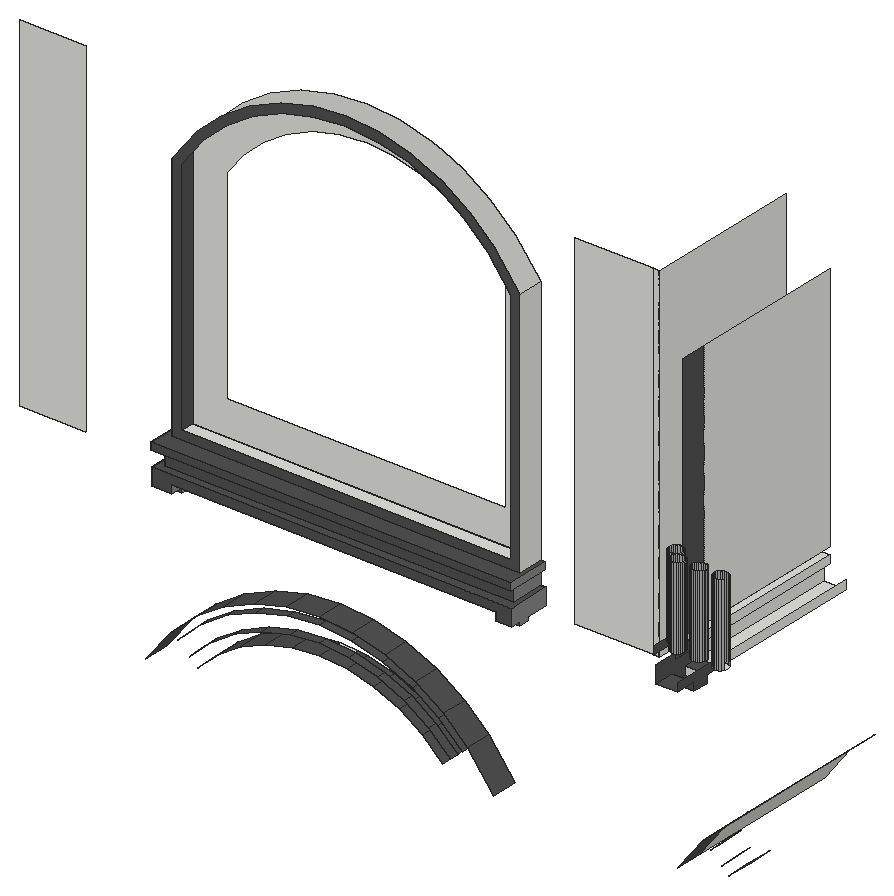
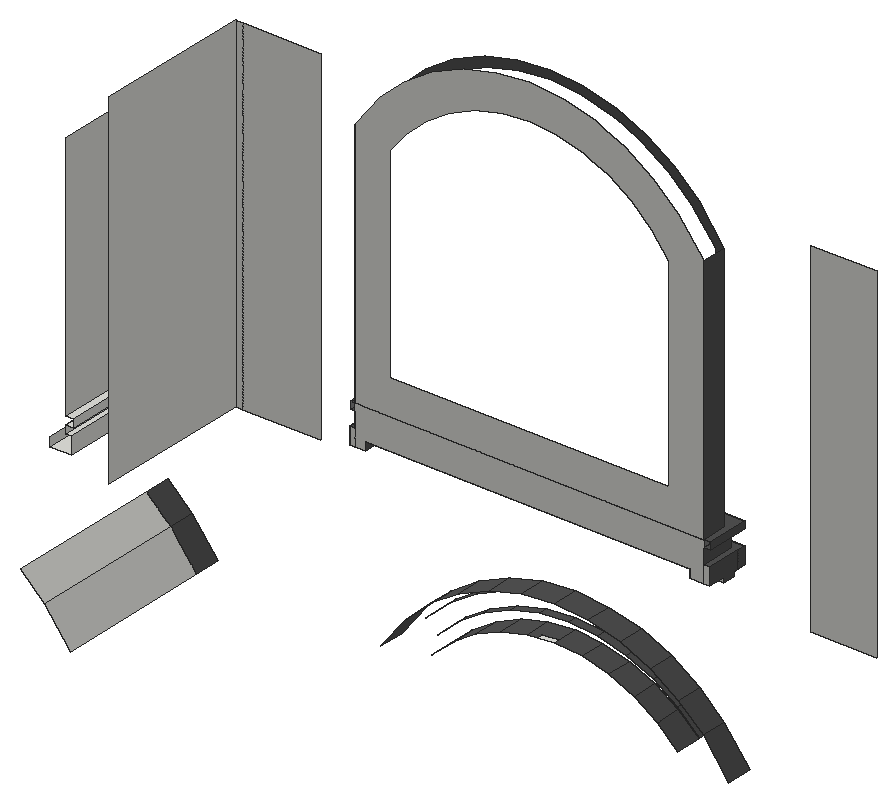
# SketchUp Ruby script. Lengths in inches.
U = 1.inch
M = Sketchup.active_model
def pt(a) = Geom::Point3d.new(a.map { |v| v * U })
def face(e, loops, mat)
  f = e.add_face(loops[0].map { |a| pt(a) })
  loops[1..].each { |l| e.add_face(l.map { |a| pt(a) }).erase! }
  f.material = f.back_material = mat if mat
  f
end
# faces: each face lists its corners as indices into pts; further lists are holes
def faces(e, pts, list, mat = nil) = list.each { |f| face(e, (f[0].is_a?(Array) ? f : [f]).map { |l| l.map { |i| pts[i] } }, mat) }
# xy, xz, yz: faces in a plane at the given z, y or x. An outline is a flat list of corners, or four numbers for a rectangle; further outlines are holes
def ring(l) = l.size == 4 ? [[l[0], l[1]], [l[2], l[1]], [l[2], l[3]], [l[0], l[3]]] : l.each_slice(2).to_a
def flat(e, list, mat, &to3) = list.each { |f| face(e, (f[0].is_a?(Array) ? f : [f]).map { |l| ring(l).map { |u, v| to3.(u, v) } }, mat) }
def xy(e, z, list, mat = nil) = flat(e, list, mat) { |x, y| [x, y, z] }
def xz(e, y, list, mat = nil) = flat(e, list, mat) { |x, z| [x, y, z] }
def yz(e, x, list, mat = nil) = flat(e, list, mat) { |y, z| [x, y, z] }
def lines(e, pts, list) = list.each { |a, b| e.add_line(pt(pts[a]), pt(pts[b])) }
# prism: a flat outline (further loops are holes) pulled along v
def prism(e, loops, v, mat = nil)
  f = face(e, loops, mat); d = Geom::Vector3d.new(v.map { |x| x * U })
  f.pushpull(f.normal.samedirection?(d) ? d.length : -d.length)
end
def box(e, o, s, mat = nil) = prism(e, [[o, [o[0] + s[0], o[1], o[2]], [o[0] + s[0], o[1] + s[1], o[2]], [o[0], o[1] + s[1], o[2]]]], [0, 0, s[2]], mat)
def at(x, y, z, deg = 0) = Geom::Transformation.translation(pt([x, y, z])) * Geom::Transformation.rotation(ORIGIN, Z_AXIS, deg.degrees)
def axes(o, x, y, z) = Geom::Transformation.new([*x, 0, *y, 0, *z, 0, *pt(o).to_a, 1])
def part(name) = M.definitions.add(name)
# library, detail: a bought-in or finely detailed component or shape, given as its bounding box
def library(name, o, s) = part(name).tap { |d| box(d.entities, o, s) }
def detail(e, o, s) = box(e.add_group.entities, o, s)
def put(e, d, t, mat = nil) = e.add_instance(d, t).tap { |i| i.material = mat if mat }
def group(e, t, mat = nil) = e.add_group.tap { |g| g.transformation = t; g.material = mat if mat }.entities
root = M.entities
M.materials.add("[0132_LightGray]").color = [169, 169, 169]
M.materials.add("[0133_Gray]").color = [135, 135, 135]
M.materials.add("[0135_DarkGray]").color = [81, 81, 81]
xy(root,480.35,[[62.57,39.32,69.5625,43.6875]],"[0135_DarkGray]")
xy(root,480.91,[[181.99,38.25,187.51,42]],"[0135_DarkGray]")
xy(root,481.53,[[240.07,38.6875,247.74,44.12]],"[0135_DarkGray]")
xy(root,481.97,[[62.57,34.6875,69.5625,39.32],[181.99,34.6875,187.51,38.25],[181.99,42,187.51,49.6875],[62.57,43.6875,69.5625,49.6875]],"[0135_DarkGray]")
xy(root,484.28,[[240.07,49.6875,247.74,104.375]])
xy(root,484.28,[[240.07,31.6875,247.74,38.6875],[240.07,44.12,247.74,49.6875]],"[0135_DarkGray]")
xy(root,484.97,[[69.5625,34.6875,181.99,49.6875]],"[0135_DarkGray]")
xy(root,487.85,[[62.57,34.6875,187.51,34.6875,187.51,49.6875,185.82,49.6875,185.82,37.6875,64.89,37.6875,64.89,49.6875,62.57,49.6875]],"[0135_DarkGray]")
xy(root,490.18,[[240.07,49.6875,242.14,104.375]])
xy(root,493.07,[[239.45,49.6875,242.14,104.375]])
xy(root,493.17,[[62.39,34.6875,62.39,49.6875,64.89,49.6875,64.89,37.6875,185.82,37.6875,185.82,49.6875,187.14,49.6875,187.14,34.6875]],"[0135_DarkGray]")
xy(root,495.66,[[245.54,31.88,244.91,31.96,244.32,32.21,243.82,32.6,243.43,33.1,243.18,33.6875,243.1,34.32,243.18,34.95,243.43,35.54,243.82,36.04,244.32,36.43,244.91,36.67,245.54,36.76,246.17,36.67,246.76,36.43,247.26,36.04,247.65,35.54,247.89,34.95,247.98,34.32,247.89,33.6875,247.65,33.1,247.26,32.6,246.76,32.21,246.17,31.96],[252.98,31.88,252.35,31.96,251.76,32.21,251.25,32.6,250.87,33.1,250.62,33.6875,250.54,34.32,250.62,34.95,250.87,35.54,251.25,36.04,251.76,36.43,252.35,36.67,252.98,36.76,253.61,36.67,254.2,36.43,254.7,36.04,255.09,35.54,255.33,34.95,255.41,34.32,255.33,33.6875,255.09,33.1,254.7,32.6,254.2,32.21,253.61,31.96],[260.41,31.88,259.78,31.96,259.2,32.21,258.69,32.6,258.3,33.1,258.06,33.6875,257.98,34.32,258.06,34.95,258.3,35.54,258.69,36.04,259.2,36.43,259.78,36.67,260.41,36.76,261.04,36.67,261.63,36.43,262.14,36.04,262.53,35.54,262.77,34.95,262.85,34.32,262.77,33.6875,262.53,33.1,262.14,32.6,261.63,32.21,261.04,31.96],[64.89,40.6875,185.57,49.6875],[239.45,49.6875,242.14,104.375]])
xy(root,495.66,[[62.39,34.6875,187.14,34.6875,187.14,49.6875,185.57,49.6875,185.57,40.6875,64.89,40.6875,64.89,49.6875,62.39,49.6875]],"[0135_DarkGray]")
xz(root,34.6875,[[62.57,481.97,69.5625,481.97,69.5625,484.97,181.99,484.97,181.99,481.97,187.51,481.97,187.51,487.85,62.57,487.85],[62.39,493.17,187.14,495.66]],"[0135_DarkGray]")
xz(root,37.6875,[[64.89,487.85,185.82,493.17]],"[0135_DarkGray]")
xz(root,38.25,[[181.99,480.91,187.51,481.97]],"[0135_DarkGray]")
xz(root,38.6875,[[240.07,481.53,247.74,484.28]],"[0135_DarkGray]")
xz(root,39.32,[[62.57,480.35,69.5625,481.97]],"[0135_DarkGray]")
xz(root,40.6875,[[[64.89,495.66,185.57,495.66,185.57,582.07,176.65,593.68,168.18,601.54,158.52,607.9,151.56,610.98,147.95,612.57,136.75,615.43,125.23,616.39,113.71,615.43,102.51,612.57,98.9,610.98,91.93,607.9,82.28,601.54,73.8125,593.68,64.89,582.07],[67.9,498.68,67.9,581.05,76.05,591.64,84.15,599.16,93.38,605.24,100.12,608.22,103.5,609.71,114.21,612.4375,125.23,613.36,136.25,612.4375,146.96,609.71,150.34,608.22,157.07,605.24,166.31,599.16,174.41,591.64,182.55,581.05,182.55,498.68]]],"[0135_DarkGray]")
xz(root,42,[[181.99,480.91,187.51,481.97]])
xz(root,43.6875,[[62.57,480.35,69.5625,481.97]])
xz(root,44.12,[[240.07,481.53,247.74,484.28]])
xz(root,49.6875,[[4.9375,480,27.68,600],[197.35,480,224.47,600],[224.47,480,226.6,600],[226.6,480,227.04,600],[62.57,481.97,64.89,487.85],
  [64.89,481.97,69.5625,481.97,69.5625,484.97,181.99,484.97,181.99,481.97,185.82,481.97,185.82,495.66,64.89,495.66],[185.82,481.97,187.51,487.85],[[64.89,495.66,185.57,495.66,185.57,582.07,176.65,593.68,168.18,601.54,158.52,607.9,151.56,610.98,147.95,612.57,136.75,615.43,125.23,616.39,113.71,615.43,102.51,612.57,98.9,610.98,91.93,607.9,82.28,601.54,73.8125,593.68,64.89,582.07],[76.89,507.66,76.89,577.99,82.71,585.57,89.72,592.07,97.7,597.33,103.75,600,106.44,601.19,115.7,603.55,122.29,604.1,125.23,604.35,134.75,603.55,144.02,601.19,146.71,600,152.76,597.33,160.74,592.07,167.74,585.57,173.57,577.99,173.57,507.66]]])
yz(root,62.39,[[34.6875,493.17,49.6875,495.66]],"[0135_DarkGray]")
yz(root,62.57,[[39.32,480.35,39.32,481.97,37.6875,481.97,37.6875,487.85,49.6875,487.85,49.6875,481.97,43.6875,481.97,43.6875,480.35],[34.6875,481.97,37.6875,487.85]],"[0135_DarkGray]")
yz(root,64.89,[[37.6875,487.85,49.6875,493.17],[40.6875,495.66,49.6875,582.07]],"[0135_DarkGray]")
yz(root,69.5625,[[39.32,480.35,43.6875,480.35,43.6875,481.97,49.6875,481.97,49.6875,484.97,34.6875,484.97,34.6875,481.97,39.32,481.97]],"[0133_Gray]")
yz(root,181.99,[[38.25,480.91,38.25,481.97,34.6875,481.97,34.6875,484.97,49.6875,484.97,49.6875,481.97,42,481.97,42,480.91]],"[0135_DarkGray]")
yz(root,185.57,[[40.6875,495.66,49.6875,582.07]])
yz(root,185.82,[[37.6875,487.85,49.6875,493.17]],"[0133_Gray]")
yz(root,187.14,[[34.6875,493.17,49.6875,495.66]],"[0133_Gray]")
yz(root,187.51,[[38.25,480.91,42,480.91,42,481.97,49.6875,481.97,49.6875,487.85,34.6875,487.85,34.6875,481.97,38.25,481.97]],"[0133_Gray]")
yz(root,227.04,[[49.6875,480,104.375,600]])
yz(root,239.45,[[49.6875,493.07,104.375,495.66]])
yz(root,239.45,[[31.6875,493.07,49.6875,495.66]],"[0135_DarkGray]")
yz(root,240.07,[[49.6875,484.28,104.375,490.18]])
yz(root,240.07,[[38.6875,481.53,38.6875,484.28,31.6875,484.28,31.6875,490.18,49.6875,490.18,49.6875,484.28,44.12,484.28,44.12,481.53]],"[0135_DarkGray]")
yz(root,242.14,[[49.6875,490.18,104.375,493.07],[49.6875,495.66,104.375,582.07]])
yz(root,242.14,[[37.6875,490.18,49.6875,493.07],[40.6875,495.66,49.6875,582.07]],"[0135_DarkGray]")
yz(root,247.74,[[49.6875,484.28,104.375,487.28]])
yz(root,247.74,[[38.6875,481.53,44.12,481.53,44.12,484.28,49.6875,484.28,49.6875,487.28,31.6875,487.28,31.6875,484.28,38.6875,484.28]],"[0135_DarkGray]")
p = [[64.875,49.6875,434.86],[55.95,49.6875,423.26],[55.95,40.6875,423.26],[64.875,40.6875,434.86],[176.64,49.6875,423.26],[167.71,49.6875,434.86],
  [167.71,40.6875,434.86],[176.64,40.6875,423.26],[249.375,49.6875,434.86],[240.45,49.6875,423.26],[240.45,40.6875,423.26],[249.375,40.6875,434.86],
  [240.45,104.375,423.26],[249.375,104.375,434.86],[73.78,49.6875,426.75],[80.78,49.6875,433.26],[80.78,40.6875,433.26],[73.78,40.6875,426.75],
  [151.8,49.6875,433.26],[158.81,49.6875,426.75],[158.81,40.6875,426.75],[151.8,40.6875,433.26],[258.28,49.6875,426.75],[265.28,49.6875,433.26],
  [265.28,40.6875,433.26],[258.28,40.6875,426.75],[263.08,43.6875,436.06],[255.65,43.6875,429.15],[255.65,40.6875,429.15],[263.08,40.6875,436.06],
  [78.4,43.6875,436.29],[70.93,43.6875,429.35],[70.93,40.6875,429.35],[78.4,40.6875,436.29],[161.65,43.6875,429.35],[154.18,43.6875,436.29],
  [154.18,40.6875,436.29],[161.65,40.6875,429.35],[251.82,43.6875,432.64],[259.88,43.6875,440.13],[259.88,40.6875,440.13],[251.82,40.6875,432.64],
  [66.8,43.6875,433.11],[74.95,43.6875,440.68],[74.95,40.6875,440.68],[66.8,40.6875,433.11],[157.63,43.6875,440.68],[165.78,43.6875,433.11],
  [165.78,40.6875,433.11],[157.63,40.6875,440.68],[88.76,49.6875,438.52],[88.76,40.6875,438.52],[143.82,49.6875,438.52],[143.82,40.6875,438.52],
  [73.34,49.6875,442.73],[73.34,40.6875,442.73],[159.24,49.6875,442.73],[159.24,40.6875,442.73],[257.84,49.6875,442.73],[257.84,40.6875,442.73],
  [257.84,104.375,442.73],[86.92,43.6875,441.9],[86.92,40.6875,441.9],[145.66,43.6875,441.9],[145.66,40.6875,441.9],[97.5,49.6875,442.38],
  [97.5,40.6875,442.38],[135.08,49.6875,442.38],[135.08,40.6875,442.38],[84.25,43.6875,446.8],[84.25,40.6875,446.8],[148.34,43.6875,446.8],
  [148.34,40.6875,446.8],[96.25,43.6875,446.02],[96.25,40.6875,446.02],[136.34,43.6875,446.02],[136.34,40.6875,446.02],[106.77,49.6875,444.74],
  [106.77,40.6875,444.74],[125.82,49.6875,444.74],[125.82,40.6875,444.74],[83,49.6875,449.09],[83,40.6875,449.09],[149.59,49.6875,449.09],
  [149.59,40.6875,449.09],[116.29,49.6875,445.53],[116.29,47.6875,445.53],[116.29,40.6875,445.53],[122.29,47.6875,445.03],[122.29,49.6875,445.03],
  [106.13,43.6875,448.53],[106.13,40.6875,448.53],[126.45,43.6875,448.53],[126.45,40.6875,448.53],[94.42,43.6875,451.29],[94.42,40.6875,451.29],
  [138.16,43.6875,451.29],[138.16,40.6875,451.29],[116.29,43.6875,449.38],[116.29,40.6875,449.38],[93.57,49.6875,453.76],[93.57,40.6875,453.76],
  [139.01,49.6875,453.76],[139.01,40.6875,453.76],[105.2,43.6875,454.04],[105.2,40.6875,454.04],[127.38,43.6875,454.04],[127.38,40.6875,454.04],
  [104.77,49.6875,456.61],[104.77,40.6875,456.61],[127.8125,49.6875,456.61],[127.8125,40.6875,456.61],[116.29,43.6875,454.96],[116.29,40.6875,454.96],
  [116.29,49.6875,457.57],[116.29,40.6875,457.57],[244.91,31.96,495.66],[245.54,31.88,495.66],[245.54,31.88,523.91],[244.91,31.96,523.91],
  [246.17,31.96,495.66],[246.17,31.96,523.91],[252.35,31.96,495.66],[252.98,31.88,495.66],[252.98,31.88,523.91],[252.35,31.96,523.91],
  [253.61,31.96,495.66],[253.61,31.96,523.91],[259.78,31.96,495.66],[260.41,31.88,495.66],[260.41,31.88,523.91],[259.78,31.96,523.91],
  [261.04,31.96,495.66],[261.04,31.96,523.91],[244.32,32.21,495.66],[244.32,32.21,523.91],[246.76,32.21,495.66],[246.76,32.21,523.91],
  [251.76,32.21,495.66],[251.76,32.21,523.91],[254.2,32.21,495.66],[254.2,32.21,523.91],[259.2,32.21,495.66],[259.2,32.21,523.91],
  [261.63,32.21,495.66],[261.63,32.21,523.91],[243.82,32.6,495.66],[243.82,32.6,523.91],[247.26,32.6,495.66],[247.26,32.6,523.91],
  [251.25,32.6,495.66],[251.25,32.6,523.91],[254.7,32.6,495.66],[254.7,32.6,523.91],[258.69,32.6,495.66],[258.69,32.6,523.91],
  [262.14,32.6,495.66],[262.14,32.6,523.91],[243.43,33.1,495.66],[243.43,33.1,523.91],[247.65,33.1,495.66],[247.65,33.1,523.91],
  [250.87,33.1,495.66],[250.87,33.1,523.91],[255.09,33.1,495.66],[255.09,33.1,523.91],[258.3,33.1,495.66],[258.3,33.1,523.91],
  [262.53,33.1,495.66],[262.53,33.1,523.91],[243.18,33.6875,495.66],[243.18,33.6875,523.91],[247.89,33.6875,495.66],[247.89,33.6875,523.91],
  [250.62,33.6875,495.66],[250.62,33.6875,523.91],[255.33,33.6875,495.66],[255.33,33.6875,523.91],[258.06,33.6875,495.66],[258.06,33.6875,523.91],
  [243.1,34.32,495.66],[243.1,34.32,523.91],[247.98,34.32,495.66],[247.98,34.32,523.91],[250.54,34.32,495.66],[250.54,34.32,523.91],
  [255.41,34.32,495.66],[255.41,34.32,523.91],[257.98,34.32,495.66],[257.98,34.32,523.91],[243.18,34.95,495.66],[243.18,34.95,523.91],
  [247.89,34.95,495.66],[247.89,34.95,523.91],[250.62,34.95,495.66],[250.62,34.95,523.91],[255.33,34.95,495.66],[255.33,34.95,523.91],
  [258.06,34.95,495.66],[258.06,34.95,523.91],[243.43,35.54,495.66],[243.43,35.54,523.91],[247.65,35.54,495.66],[247.65,35.54,523.91],
  [250.87,35.54,495.66],[250.87,35.54,523.91],[255.09,35.54,495.66],[255.09,35.54,523.91],[258.3,35.54,495.66],[258.3,35.54,523.91],
  [243.82,36.04,495.66],[243.82,36.04,523.91],[247.26,36.04,495.66],[247.26,36.04,523.91],[251.25,36.04,495.66],[251.25,36.04,523.91],
  [254.7,36.04,495.66],[254.7,36.04,523.91],[258.69,36.04,495.66],[258.69,36.04,523.91],[240.74,35.88,495.66],[241.33,35.64,495.66],
  [241.33,35.64,523.91],[240.74,35.88,523.91],[241.96,35.55,495.66],[241.96,35.55,523.91],[242.59,35.64,495.66],[242.59,35.64,523.91],
  [243.18,35.88,495.66],[243.18,35.88,523.91],[240.24,36.27,495.66],[240.24,36.27,523.91],[243.6875,36.27,495.66],[243.6875,36.27,523.91],
  [244.32,36.43,495.66],[244.32,36.43,523.91],[246.76,36.43,495.66],[246.76,36.43,523.91],[251.76,36.43,495.66],[251.76,36.43,523.91],
  [254.2,36.43,495.66],[254.2,36.43,523.91],[259.2,36.43,495.66],[259.2,36.43,523.91],[262.14,36.04,495.66],[261.63,36.43,495.66],
  [261.63,36.43,523.91],[262.14,36.04,523.91],[239.85,36.77,495.66],[239.85,36.77,523.91],[244.07,36.77,495.66],[244.07,36.77,523.91],
  [244.91,36.67,495.66],[244.91,36.67,523.91],[246.17,36.67,495.66],[246.17,36.67,523.91],[252.35,36.67,495.66],[252.35,36.67,523.91],
  [253.61,36.67,495.66],[253.61,36.67,523.91],[259.78,36.67,495.66],[259.78,36.67,523.91],[261.04,36.67,495.66],[261.04,36.67,523.91],
  [245.54,36.76,495.66],[245.54,36.76,523.91],[252.98,36.76,495.66],[252.98,36.76,523.91],[260.41,36.76,495.66],[260.41,36.76,523.91],
  [239.61,37.36,495.66],[239.61,37.36,523.91],[244.32,37.36,495.66],[244.32,37.36,523.91],[239.52,37.99,495.66],[239.52,37.99,523.91],
  [244.4,37.99,495.66],[244.4,37.99,523.91],[239.61,38.62,495.66],[239.61,38.62,523.91],[244.32,38.62,495.66],[244.32,38.62,523.91],
  [239.85,39.21,495.66],[239.85,39.21,523.91],[244.07,39.21,495.66],[244.07,39.21,523.91],[240.24,39.71,495.66],[240.24,39.71,523.91],
  [243.6875,39.71,495.66],[243.6875,39.71,523.91],[240.74,40.1,495.66],[240.74,40.1,523.91],[243.18,40.1,495.66],[243.18,40.1,523.91],
  [241.33,40.34,495.66],[241.33,40.34,523.91],[242.59,40.34,495.66],[242.59,40.34,523.91],[241.96,40.43,495.66],[241.96,40.43,523.91],
  [64.89,37.6875,484.97],[64.89,37.6875,487.85],[185.82,37.6875,487.85],[185.82,37.6875,484.97],[64.89,37.6875,493.17],[64.89,37.6875,495.66]]
faces(root,p,[[0,1,2,3],[4,5,6,7],[8,9,10,11],[14,15,16,17],[18,19,20,21],[22,23,24,25],[26,27,28,29],[30,31,32,33],
  [34,35,36,37],[38,39,40,41],[42,43,44,45],[46,47,48,49],[15,50,51,16],[52,18,21,53],[54,0,3,55],[5,56,57,6],
  [58,8,11,59],[61,30,33,62],[35,63,64,36],[50,65,66,51],[67,52,53,68],[43,69,70,44],[71,46,49,72],[73,61,62,74],
  [63,75,76,64],[65,77,78,66],[79,67,68,80],[81,54,55,82],[56,83,84,57],[77,85,86,87,78],[87,86,88,89,79,80],[90,73,74,91],
  [75,92,93,76],[69,94,95,70],[96,71,72,97],[98,90,91,99],[92,98,99,93],[100,81,82,101],[83,102,103,84],[94,104,105,95],
  [106,96,97,107],[108,100,101,109],[102,110,111,103],[104,112,113,105],[112,106,107,113],[114,108,109,115],[110,114,115,111]],"[0135_DarkGray]")
faces(root,p,[[8,9,12,13],[58,8,13,60],[85,89,88,86]])
faces(root,p,[[116,117,118,119],[117,120,121,118],[122,123,124,125],[123,126,127,124],[128,129,130,131],[129,132,133,130],[134,116,119,135],[120,136,137,121],
  [138,122,125,139],[126,140,141,127],[142,128,131,143],[132,144,145,133],[146,134,135,147],[136,148,149,137],[150,138,139,151],[140,152,153,141],
  [154,142,143,155],[144,156,157,145],[158,146,147,159],[148,160,161,149],[162,150,151,163],[152,164,165,153],[166,154,155,167],[156,168,169,157],
  [170,158,159,171],[160,172,173,161],[174,162,163,175],[164,176,177,165],[178,166,167,179],[180,170,171,181],[172,182,183,173],[184,174,175,185],
  [176,186,187,177],[188,178,179,189],[190,180,181,191],[182,192,193,183],[194,184,185,195],[186,196,197,187],[198,188,189,199],[200,190,191,201],
  [192,202,203,193],[204,194,195,205],[196,206,207,197],[208,198,199,209],[210,200,201,211],[202,212,213,203],[214,204,205,215],[206,216,217,207],
  [218,208,209,219],[220,221,222,223],[221,224,225,222],[224,226,227,225],[226,228,229,227],[230,220,223,231],[228,232,233,229],[234,210,211,235],
  [212,236,237,213],[238,214,215,239],[216,240,241,217],[242,218,219,243],[244,245,246,247],[248,230,231,249],[232,250,251,233],[252,234,235,253],
  [236,254,255,237],[256,238,239,257],[240,258,259,241],[260,242,243,261],[245,262,263,246],[264,252,253,265],[254,264,265,255],[266,256,257,267],
  [258,266,267,259],[268,260,261,269],[262,268,269,263],[270,248,249,271],[250,272,273,251],[274,270,271,275],[272,276,277,273],[278,274,275,279],
  [276,280,281,277],[282,278,279,283],[280,284,285,281],[286,282,283,287],[284,288,289,285],[290,286,287,291],[288,292,293,289],[294,290,291,295],
  [292,296,297,293],[298,294,295,299],[296,298,299,297]],"[0132_LightGray]")
lines(root,p,[[300,301],[302,303],[304,305]])
